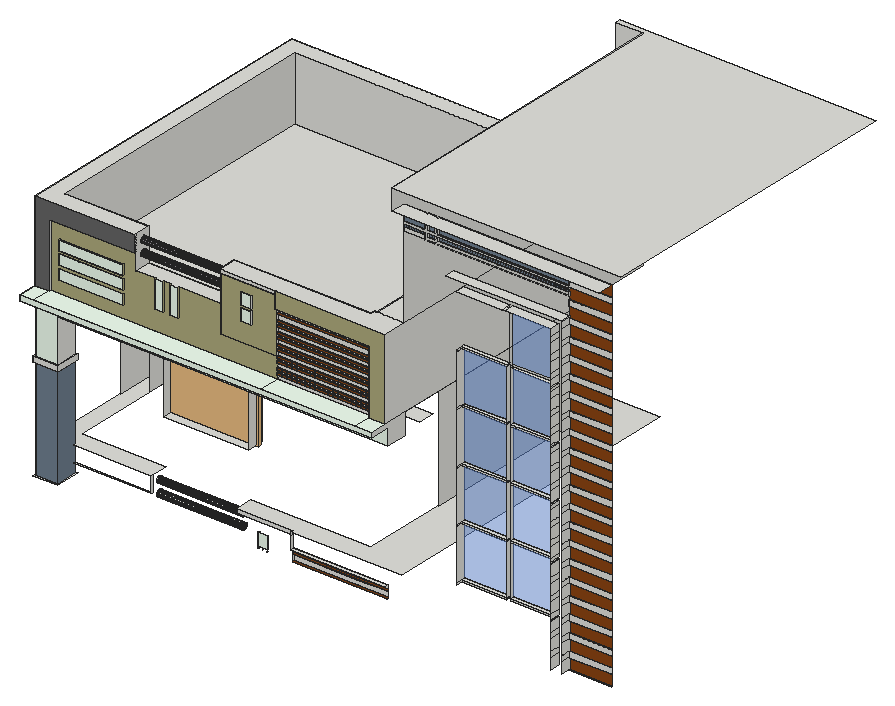
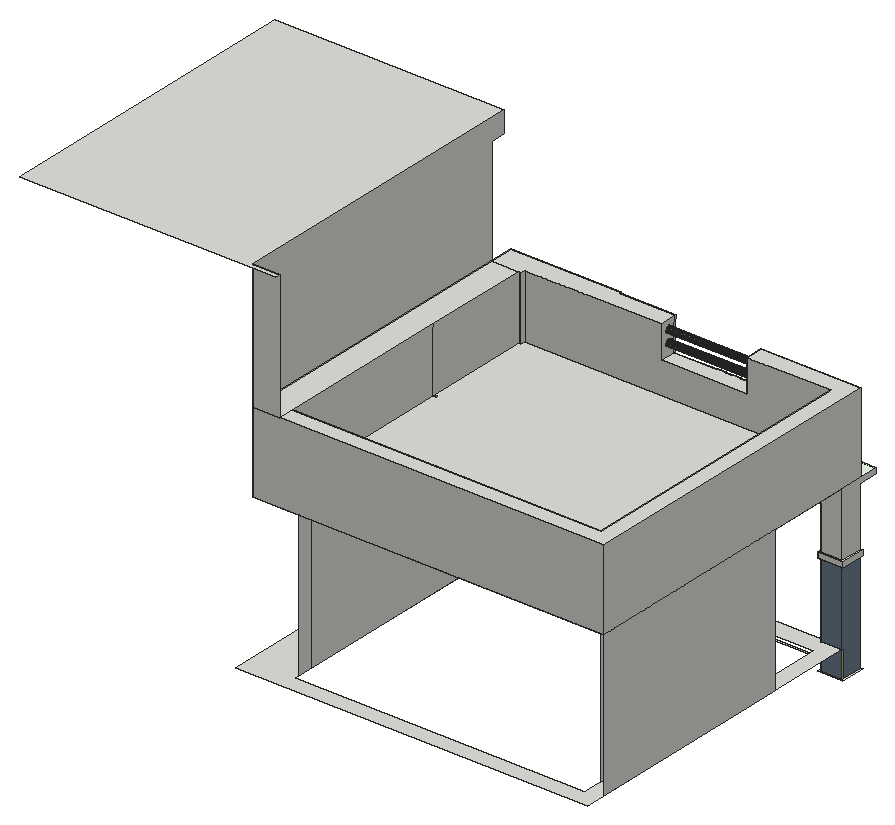
# SketchUp Ruby script. Lengths in inches.
U = 1.inch
M = Sketchup.active_model
def pt(a) = Geom::Point3d.new(a.map { |v| v * U })
def face(e, loops, mat)
  f = e.add_face(loops[0].map { |a| pt(a) })
  loops[1..].each { |l| e.add_face(l.map { |a| pt(a) }).erase! }
  f.material = f.back_material = mat if mat
  f
end
# faces: each face lists its corners as indices into pts; further lists are holes
def faces(e, pts, list, mat = nil) = list.each { |f| face(e, (f[0].is_a?(Array) ? f : [f]).map { |l| l.map { |i| pts[i] } }, mat) }
# xy, xz, yz: faces in a plane at the given z, y or x. An outline is a flat list of corners, or four numbers for a rectangle; further outlines are holes
def ring(l) = l.size == 4 ? [[l[0], l[1]], [l[2], l[1]], [l[2], l[3]], [l[0], l[3]]] : l.each_slice(2).to_a
def flat(e, list, mat, &to3) = list.each { |f| face(e, (f[0].is_a?(Array) ? f : [f]).map { |l| ring(l).map { |u, v| to3.(u, v) } }, mat) }
def xy(e, z, list, mat = nil) = flat(e, list, mat) { |x, y| [x, y, z] }
def xz(e, y, list, mat = nil) = flat(e, list, mat) { |x, z| [x, y, z] }
def yz(e, x, list, mat = nil) = flat(e, list, mat) { |y, z| [x, y, z] }
def lines(e, pts, list) = list.each { |a, b| e.add_line(pt(pts[a]), pt(pts[b])) }
# prism: a flat outline (further loops are holes) pulled along v
def prism(e, loops, v, mat = nil)
  f = face(e, loops, mat); d = Geom::Vector3d.new(v.map { |x| x * U })
  f.pushpull(f.normal.samedirection?(d) ? d.length : -d.length)
end
def box(e, o, s, mat = nil) = prism(e, [[o, [o[0] + s[0], o[1], o[2]], [o[0] + s[0], o[1] + s[1], o[2]], [o[0], o[1] + s[1], o[2]]]], [0, 0, s[2]], mat)
def at(x, y, z, deg = 0) = Geom::Transformation.translation(pt([x, y, z])) * Geom::Transformation.rotation(ORIGIN, Z_AXIS, deg.degrees)
def axes(o, x, y, z) = Geom::Transformation.new([*x, 0, *y, 0, *z, 0, *pt(o).to_a, 1])
def part(name) = M.definitions.add(name)
# library, detail: a bought-in or finely detailed component or shape, given as its bounding box
def library(name, o, s) = part(name).tap { |d| box(d.entities, o, s) }
def detail(e, o, s) = box(e.add_group.entities, o, s)
def put(e, d, t, mat = nil) = e.add_instance(d, t).tap { |i| i.material = mat if mat }
def group(e, t, mat = nil) = e.add_group.tap { |g| g.transformation = t; g.material = mat if mat }.entities
root = M.entities
M.materials.add("Teddy_Bracelet").color = [145, 141, 147]
M.materials.add("[0043_SaddleBrown]").color = [139, 69, 19]
M.materials.add("[0047_Khaki]").color = [198, 190, 116]
M.materials.add("[0048_PaleGoldenrod]1").color = [175, 171, 125]
M.materials.add("[0066_Honeydew]").color = [240, 255, 240]
M.materials.add("[0111_SlateGray]").color = [112, 128, 144]
M.materials.add("[0134_DimGray]").color = [102, 102, 102]
M.materials.add("[Translucent Glass Blue]").color = [100, 149, 237]
M.materials["[Translucent Glass Blue]"].alpha = 0.5
c1 = library("Double-hung window 69 in. x 58 in. triple row with mullions",[0,0,-2.625],[62,58,3.625])
c2 = part("Double-hung window assembly")
put(c2.entities,c1,axes([2046.74,517.98,-571.2],[-3.288,0,0],[0,0,3.072],[0,2.4,0]))
xy(root,149,[[136.36,47.5,172.375,48],[172.375,47.5,189.375,48]])
xy(root,149.3,[[291.09,47.5,315.09,48]])
xy(root,149.33,[[116.69,47,122.32,47.5]])
xy(root,150,[[[0,35.4375,14,49.4375],[1,36.4375,13,48.4375]],[1,36.4375,13,48.4375]])
xy(root,150,[[136.36,47.5,172.375,48],[172.375,47.5,189.375,48]],"[0043_SaddleBrown]")
xy(root,150.64,[[116.69,47,122.32,47.5]])
xy(root,153,[[136.36,47.5,172.375,48],[172.375,47.5,189.375,48]])
xy(root,154,[[136.36,47.5,172.375,48],[172.375,47.5,189.375,48]],"[0043_SaddleBrown]")
xy(root,155.45,[[291.09,47.5,315.09,48]])
xy(root,156,[[136.36,45.9375,189.375,48],[9.125,47,57.01,48]])
xy(root,157.33,[[116.69,47,122.32,47.5]])
xy(root,158.61,[[291.09,47.5,315.09,48]])
xy(root,162,[[25,95.625,73,104.625]])
xy(root,163,[[104.95,47,136.36,47.5]])
xy(root,164.77,[[291.09,47.5,315.09,48]])
xy(root,165,[[136.36,45.9375,198.375,45.9375,198.375,227.1875,1,227.1875,1,47,57.01,47,57.01,57,10,57,10,218.1875,172.375,218.1875,172.375,57,104.95,57,104.95,47,136.36,47]])
xy(root,167.92,[[291.09,47.5,315.09,48]])
xy(root,173.4,[[232.02,46,257.55,48],[259.55,46,285.09,48]])
xy(root,174.08,[[291.09,47.5,315.09,48]])
xy(root,174.4,[[232.02,46,257.55,48],[259.55,46,285.09,48]])
xy(root,177.23,[[291.09,47.5,315.09,48]])
xy(root,183.39,[[291.09,47.5,315.09,48]])
xy(root,186.55,[[291.09,47.5,315.09,48]])
xy(root,192.7,[[291.09,47.5,315.09,48]])
xy(root,195.86,[[291.09,47.5,315.09,48]])
xy(root,202.01,[[291.09,47.5,315.09,48]])
xy(root,202.68,[[232.02,46,257.55,48],[259.55,46,285.09,48]])
xy(root,203.68,[[232.02,46,257.55,47.8125],[259.55,46,285.09,48]])
xy(root,205.17,[[291.09,47.5,315.09,48]])
xy(root,207,[[0,35.4375,14,36.4375],[0,36.4375,1,49.4375],[1,36.4375,13,48.4375],[13,36.4375,14,49.4375],[1,48.4375,13,49.4375]])
xy(root,208.1875,[[25,95.625,73,104.625]])
xy(root,210,[[[0,35.4375,14,49.4375],[1,36.4375,13,48.4375]],[1,36.4375,13,48.4375],[133.23,95.625,169.23,104.625]])
xy(root,211.32,[[291.09,47.5,315.09,48]])
xy(root,214.48,[[291.09,47.5,315.09,48]])
xy(root,220.64,[[291.09,47.5,315.09,48]])
xy(root,223.79,[[291.09,47.5,315.09,48]])
xy(root,229.95,[[291.09,47.5,315.09,48]])
xy(root,231.95,[[232.02,46,257.55,47.8125],[259.55,46,285.09,48]])
xy(root,232.95,[[232.02,46,257.55,48],[259.55,46,285.09,48]])
xy(root,233.11,[[291.09,47.5,315.09,48]])
xy(root,234,[[13,36.4375,198.375,48.4375]])
xy(root,239.26,[[291.09,47.5,315.09,48]])
xy(root,242.42,[[291.09,47.5,315.09,48]])
xy(root,243,[[1,24.875,198.375,36.4375]],"[0066_Honeydew]")
xy(root,246,[[189.375,34.375,189.375,36.4375,9.125,36.4375,9.125,35.4375,1,35.4375,1,48.4375,198.375,48.4375,198.375,34.375],[1,48.4375,172.375,95.625],[172.375,48.4375,198.375,95.625],[1,95.625,172.375,95.625,172.375,104.625,10,104.625,10,206.625,172.375,206.625,172.375,215.625,1,215.625],[172.375,95.625,181.375,104.625],
  [181.375,95.625,198.375,104.625],[10,104.625,172.375,206.625],[172.375,104.625,181.375,215.625],[181.375,104.625,198.375,215.625]])
xy(root,246,[[1,24.875,9.125,35.4375],[9.125,24.875,136.36,36.4375],[136.36,24.875,189.375,36.4375],[189.375,24.875,198.375,34.375]],"[0066_Honeydew]")
xy(root,248.5,[[136.36,35.9375,172.375,36.4375],[172.375,35.9375,189.375,36.4375]])
xy(root,248.57,[[291.09,47.5,315.09,48]])
xy(root,249.5,[[136.36,35.9375,172.375,36.4375],[172.375,35.9375,189.375,36.4375]],"[0043_SaddleBrown]")
xy(root,251,[[136.36,35.9375,172.375,36.4375],[172.375,35.9375,189.375,36.4375]])
xy(root,251.73,[[291.09,47.5,315.09,48]])
xy(root,252,[[136.36,35.9375,172.375,36.4375],[172.375,35.9375,189.375,36.4375]],"[0043_SaddleBrown]")
xy(root,253.11,[[14.32,35.9375,50.14,36.4375]],"[0048_PaleGoldenrod]1")
xy(root,254.5,[[136.36,35.9375,172.375,36.4375],[172.375,35.9375,189.375,36.4375]])
xy(root,255,[[10,45.4375,181.625,45.4375,181.625,48,183,48,183,107.1875,181.375,107.1875,181.375,108,183,108,183,206.625,10,206.625],[181.375,107.1875,183,108]])
xy(root,255.5,[[136.36,35.9375,172.375,36.4375],[172.375,35.9375,189.375,36.4375]],"[0043_SaddleBrown]")
xy(root,257,[[136.36,35.9375,172.375,36.4375],[172.375,35.9375,189.375,36.4375]])
xy(root,257.375,[[68.2,35.9375,72.45,36.4375],[76.51,35.9375,80.76,36.4375]],"[0048_PaleGoldenrod]1")
xy(root,257.8125,[[104.95,35.9375,136.36,36.4375]])
xy(root,257.88,[[291.09,47.5,315.09,48]])
xy(root,258,[[136.36,35.9375,172.375,36.4375],[172.375,35.9375,189.375,36.4375]],"[0043_SaddleBrown]")
xy(root,258.61,[[14.32,35.9375,50.14,36.4375]],"[0048_PaleGoldenrod]1")
xy(root,260.5,[[136.36,35.9375,172.375,36.4375],[172.375,35.9375,189.375,36.4375]])
xy(root,260.8,[[14.32,35.9375,50.14,36.4375]],"[0048_PaleGoldenrod]1")
xy(root,261.04,[[291.09,47.5,315.09,48]])
xy(root,261.23,[[232.02,46,257.55,48],[259.55,46,285.09,48]])
xy(root,261.5,[[136.36,35.9375,172.375,36.4375],[172.375,35.9375,189.375,36.4375]],"[0043_SaddleBrown]")
xy(root,262.23,[[232.02,46,257.55,48],[259.55,46,285.09,48]])
xy(root,263,[[136.36,35.9375,172.375,36.4375],[172.375,35.9375,189.375,36.4375]])
xy(root,264,[[136.36,35.9375,172.375,36.4375],[172.375,35.9375,189.375,36.4375]],"[0043_SaddleBrown]")
xy(root,266.3,[[14.32,35.9375,50.14,36.4375]],"[0048_PaleGoldenrod]1")
xy(root,266.5,[[136.36,35.9375,172.375,36.4375],[172.375,35.9375,189.375,36.4375]])
xy(root,267.19,[[291.09,47.5,315.09,48]])
xy(root,267.5,[[136.36,35.9375,172.375,36.4375],[172.375,35.9375,189.375,36.4375]],"[0043_SaddleBrown]")
xy(root,268.05,[[14.32,35.9375,50.14,36.4375]],"[0048_PaleGoldenrod]1")
xy(root,268.64,[[116.69,35.4375,122.32,35.9375]])
xy(root,269,[[136.36,35.9375,172.375,36.4375],[172.375,35.9375,189.375,36.4375]])
xy(root,270,[[136.36,35.9375,172.375,36.4375],[172.375,35.9375,189.375,36.4375]],"[0043_SaddleBrown]")
xy(root,270.35,[[291.09,47.5,315.09,48]])
xy(root,272.5,[[136.36,35.9375,172.375,36.4375],[172.375,35.9375,189.375,36.4375]])
xy(root,272.6875,[[68.2,35.9375,72.45,35.9375,72.45,36.4375,76.51,36.4375,76.51,35.9375,80.76,35.9375,80.76,36.4375,104.95,36.4375,104.95,45.4375,57.01,45.4375,57.01,36.4375,68.2,36.4375]])
xy(root,273.5,[[136.36,35.9375,172.375,36.4375],[172.375,35.9375,189.375,36.4375]],"[0043_SaddleBrown]")
xy(root,273.55,[[14.32,35.9375,50.14,36.4375]],"[0048_PaleGoldenrod]1")
xy(root,275,[[136.36,35.9375,172.375,36.4375],[172.375,35.9375,189.375,36.4375]])
xy(root,275.33,[[116.69,35.4375,122.32,35.9375]])
xy(root,276,[[136.36,35.9375,172.375,36.4375],[172.375,35.9375,189.375,36.4375]],"[0043_SaddleBrown]")
xy(root,276.51,[[291.09,47.5,315.09,48]])
xy(root,276.64,[[116.69,35.4375,122.32,35.9375]])
xy(root,279,[[136.36,35.9375,172.375,36.4375],[172.375,35.9375,189.375,36.4375]])
xy(root,279.66,[[291.09,47.5,315.09,48]])
xy(root,280,[[136.36,35.9375,172.375,36.4375],[172.375,35.9375,189.375,36.4375]],"[0043_SaddleBrown]")
xy(root,282,[[136.36,34.375,189.375,36.4375],[9.125,35.4375,57.01,36.4375]])
xy(root,283.33,[[116.69,35.4375,122.32,35.9375]])
xy(root,285.82,[[291.09,47.5,315.09,48]])
xy(root,288.98,[[291.09,47.5,315.09,48]])
xy(root,289,[[104.95,35.4375,136.36,35.9375]])
xy(root,290.51,[[232.02,46,257.55,48],[259.55,46,285.09,48]])
xy(root,291,[[136.36,34.375,198.375,34.375,198.375,48,181.625,48,181.625,45.4375,104.95,45.4375,104.95,35.4375,136.36,35.4375],[1,35.4375,57.01,35.4375,57.01,45.4375,10,45.4375,10,206.625,183,206.625,183,215.625,1,215.625],[183,48,198.375,215.625]])
xy(root,291.51,[[232.02,46,257.55,48]])
xy(root,295.13,[[291.09,47.5,315.09,48]])
xy(root,298.29,[[291.09,47.5,315.09,48]])
xy(root,304.44,[[291.09,47.5,315.09,48]])
xy(root,307.6,[[291.09,47.5,315.09,48]])
xy(root,313.75,[[291.09,47.5,315.09,48]])
xy(root,316.91,[[291.09,47.5,315.09,48]])
xy(root,320.78,[[232.02,42.5,257.55,48],[257.55,42.5,259.55,46],[259.55,42.5,285.09,48]])
xy(root,323.06,[[291.09,47.5,315.09,48]])
xy(root,326.22,[[291.09,47.5,315.09,48]])
xy(root,326.78,[[226.02,42.5,291.09,48]])
xy(root,332.375,[[291.09,47.5,315.09,48]])
xy(root,335.53,[[291.09,47.5,315.09,48]])
xy(root,337.1875,[[212.0625,47.5,215.8125,48],[217.8125,47.5,291.09,48]])
xy(root,339.1875,[[212.0625,47.5,215.8125,48],[217.8125,47.5,291.09,48]])
xy(root,340.5,[[198.375,47.5,210.0625,48],[212.0625,47.5,215.8125,48],[217.8125,47.5,291.09,48]])
xy(root,341.6875,[[291.09,47.5,315.09,48]])
xy(root,342.5,[[198.375,47.5,210.0625,48],[212.0625,47.5,215.8125,48],[217.8125,47.5,291.09,48]])
xy(root,344.85,[[291.09,47.5,315.09,48]])
xy(root,351,[[198.375,39,198.375,48,210.0625,48,210.0625,47.5,212.0625,47.5,212.0625,48,215.8125,48,215.8125,47.5,217.8125,47.5,217.8125,48,315.09,48,315.09,39]])
xy(root,363,[[198.375,39,327,39,327,218.1875,183,218.1875,183,215.625,198.375,215.625]])
xz(root,24.875,[[1,243,198.375,246]],"[0066_Honeydew]")
xz(root,34.375,[[189.375,246,198.375,246,198.375,291,136.36,291,136.36,282,189.375,282]],"[0048_PaleGoldenrod]1")
xz(root,35.4375,[[0,207,14,210],[104.95,289,136.36,291]])
xz(root,35.4375,[[116.69,268.64,122.32,275.33],[116.69,276.64,122.32,283.33]],"[0066_Honeydew]")
xz(root,35.4375,[[1,246,9.125,246,9.125,282,57.01,282,57.01,291,1,291]],"[0134_DimGray]")
xz(root,35.9375,[[136.36,248.5,189.375,249.5],[136.36,251,189.375,252],[136.36,254.5,189.375,255.5],[136.36,257,189.375,258],[136.36,260.5,189.375,261.5],
  [136.36,263,189.375,264],[136.36,266.5,189.375,267.5],[136.36,269,189.375,270],[136.36,272.5,189.375,273.5],[136.36,275,189.375,276],
  [136.36,279,189.375,280]],"[0043_SaddleBrown]")
xz(root,35.9375,[[[104.95,257.8125,136.36,289],[116.69,276.64,122.32,283.33],[116.69,268.64,122.32,275.33]]],"[0048_PaleGoldenrod]1")
xz(root,35.9375,[[14.32,253.11,50.14,258.61],[68.2,257.375,72.45,272.6875],[76.51,257.375,80.76,272.6875],[14.32,260.8,50.14,266.3],[14.32,268.05,50.14,273.55]],"[0066_Honeydew]")
xz(root,36.4375,[[136.36,246,189.375,248.5],[136.36,249.5,189.375,251],[136.36,252,189.375,254.5],[136.36,255.5,189.375,257],[136.36,258,189.375,260.5],
  [136.36,261.5,189.375,263],[136.36,264,189.375,266.5],[136.36,267.5,189.375,269],[136.36,270,189.375,272.5],[136.36,273.5,189.375,275],
  [136.36,276,189.375,279],[136.36,280,189.375,282]])
xz(root,36.4375,[[[9.125,246,136.36,246,136.36,257.8125,104.95,257.8125,104.95,272.6875,80.76,272.6875,80.76,257.375,76.51,257.375,76.51,272.6875,72.45,272.6875,72.45,257.375,68.2,257.375,68.2,272.6875,57.01,272.6875,57.01,282,9.125,282],[14.32,268.05,50.14,273.55],[14.32,260.8,50.14,266.3],[14.32,253.11,50.14,258.61]]],"[0048_PaleGoldenrod]1")
xz(root,36.4375,[[1,210,13,210,13,234,198.375,234,198.375,243,1,243]],"[0066_Honeydew]")
xz(root,36.4375,[[1,150,13,207]],"[0111_SlateGray]")
xz(root,45.4375,[[10,255,10,291,57.01,291,57.01,272.6875,104.95,272.6875,104.95,291,181.625,291,181.625,255]])
xz(root,46,[[232.02,173.4,257.55,174.4],[259.55,173.4,285.09,174.4],[232.02,202.68,257.55,203.68],[259.55,202.68,285.09,203.68],[232.02,231.95,257.55,232.95],
  [259.55,231.95,285.09,232.95],[232.02,261.23,257.55,262.23],[259.55,261.23,285.09,262.23],[232.02,290.51,257.55,291.51]])
xz(root,47,[[104.95,163,136.36,165]])
xz(root,47,[[116.69,150.64,122.32,157.33]],"[0066_Honeydew]")
xz(root,47.5,[[291.09,155.45,315.09,158.61],[291.09,164.77,315.09,167.92],[291.09,174.08,315.09,177.23],[291.09,183.39,315.09,186.55],[291.09,192.7,315.09,195.86],
  [291.09,202.01,315.09,205.17],[291.09,211.32,315.09,214.48],[291.09,220.64,315.09,223.79],[291.09,229.95,315.09,233.11],[291.09,239.26,315.09,242.42],
  [291.09,248.57,315.09,251.73],[291.09,257.88,315.09,261.04],[291.09,267.19,315.09,270.35],[291.09,276.51,315.09,279.66],[291.09,285.82,315.09,288.98],
  [291.09,295.13,315.09,298.29],[291.09,304.44,315.09,307.6],[291.09,313.75,315.09,316.91],[291.09,323.06,315.09,326.22],[291.09,332.375,315.09,335.53],
  [291.09,341.6875,315.09,344.85]])
xz(root,47.5,[[136.36,149,189.375,150],[136.36,153,189.375,154]],"[0043_SaddleBrown]")
xz(root,47.8125,[[232.02,203.68,257.55,231.95]],"[Translucent Glass Blue]")
xz(root,48,[[136.36,150,189.375,153],[136.36,154,189.375,156],[181.625,255,183,291],[198.375,337.1875,210.0625,339.1875]])
xz(root,48,[[291.09,149.3,315.09,155.45],[291.09,158.61,315.09,164.77],[291.09,167.92,315.09,174.08],[291.09,177.23,315.09,183.39],[291.09,186.55,315.09,192.7],
  [291.09,195.86,315.09,202.01],[291.09,205.17,315.09,211.32],[291.09,214.48,315.09,220.64],[291.09,223.79,315.09,229.95],[291.09,233.11,315.09,239.26],
  [291.09,242.42,315.09,248.57],[291.09,251.73,315.09,257.88],[291.09,261.04,315.09,267.19],[291.09,270.35,315.09,276.51],[291.09,279.66,315.09,285.82],
  [291.09,288.98,315.09,295.13],[291.09,298.29,315.09,304.44],[291.09,307.6,315.09,313.75],[291.09,316.91,315.09,323.06],[291.09,326.22,315.09,332.375],
  [291.09,335.53,315.09,341.6875],[291.09,344.85,315.09,351]],"[0043_SaddleBrown]")
xz(root,48,[[198.375,339.1875,210.0625,340.5],[212.0625,339.1875,215.8125,340.5],[217.8125,339.1875,291.09,340.5],[198.375,342.5,210.0625,351],[212.0625,342.5,215.8125,351],
  [217.8125,342.5,291.09,351]],"[0111_SlateGray]")
xz(root,48,[[232.02,174.4,257.55,202.68],[259.55,174.4,285.09,202.68],[259.55,203.68,285.09,231.95],[232.02,232.95,257.55,261.23],[259.55,232.95,285.09,261.23],
  [232.02,262.23,257.55,290.51],[259.55,262.23,285.09,290.51],[259.55,291.51,285.09,320.78]],"[Translucent Glass Blue]")
xz(root,48.4375,[[1,210,1,246,198.375,246,198.375,234,13,234,13,210]])
xz(root,48.4375,[[1,150,13,207]],"[0111_SlateGray]")
xz(root,49.4375,[[0,207,14,210]])
xz(root,206.625,[[10,255,183,291]])
xz(root,215.625,[[1,246,198.375,291],[183,291,198.375,363]])
yz(root,0,[[35.4375,207,49.4375,210]])
yz(root,1,[[95.625,165,215.625,246],[36.4375,210,36.4375,243,24.875,243,24.875,246,48.4375,246,48.4375,210],[35.4375,246,215.625,291]])
yz(root,1,[[47,150,48.4375,165]],"[0047_Khaki]")
yz(root,1,[[36.4375,150,36.4375,207,48.4375,207,48.4375,165,47,165,47,150]],"[0111_SlateGray]")
yz(root,9.125,[[35.4375,246,36.4375,282]])
yz(root,10,[[104.625,165,206.625,246],[45.4375,255,206.625,291]])
yz(root,13,[[36.4375,210,48.4375,234]])
yz(root,13,[[36.4375,150,48.4375,207]],"[0111_SlateGray]")
yz(root,14,[[35.4375,207,49.4375,210]])
yz(root,14.32,[[35.9375,253.11,36.4375,258.61],[35.9375,260.8,36.4375,266.3],[35.9375,268.05,36.4375,273.55]],"[0048_PaleGoldenrod]1")
yz(root,25,[[95.625,162,104.625,208.1875]])
yz(root,50.14,[[35.9375,253.11,36.4375,258.61],[35.9375,260.8,36.4375,266.3],[35.9375,268.05,36.4375,273.55]],"[0048_PaleGoldenrod]1")
yz(root,57.01,[[47,156,48,165],[[36.4375,272.6875,45.4375,291],[41.02,284.88,40.58,284.94,40.18,285.11,39.83,285.38,39.56,285.73,39.39,286.13,39.33,286.57,39.39,287.01,39.56,287.41,39.83,287.76,40.18,288.03,40.58,288.2,41.02,288.26,41.46,288.2,41.86,288.03,42.21,287.76,42.48,287.41,42.65,287.01,42.71,286.57,42.65,286.13,42.48,285.73,42.21,285.38,41.86,285.11,41.46,284.94],[41.02,278.13,40.58,278.19,40.18,278.36,39.83,278.63,39.56,278.98,39.39,279.38,39.33,279.82,39.39,280.26,39.56,280.66,39.83,281.01,40.18,281.28,40.58,281.45,41.02,281.51,41.46,281.45,41.86,281.28,42.21,281.01,42.48,280.66,42.65,280.26,42.71,279.82,42.65,279.38,42.48,278.98,42.21,278.63,41.86,278.36,41.46,278.19]],[35.4375,282,36.4375,291]])
yz(root,68.2,[[35.9375,257.375,36.4375,272.6875]],"[0048_PaleGoldenrod]1")
yz(root,72.45,[[35.9375,257.375,36.4375,272.6875]],"[0048_PaleGoldenrod]1")
yz(root,73,[[95.625,162,104.625,208.1875]])
yz(root,76.51,[[35.9375,257.375,36.4375,272.6875]],"[0048_PaleGoldenrod]1")
yz(root,80.76,[[35.9375,257.375,36.4375,272.6875]],"[0048_PaleGoldenrod]1")
yz(root,104.95,[[47,163,48,165],[35.9375,257.8125,36.4375,272.6875],[35.9375,272.6875,36.4375,289],[[36.4375,272.6875,45.4375,291],[41.02,284.88,41.46,284.94,41.86,285.11,42.21,285.38,42.48,285.73,42.65,286.13,42.71,286.57,42.65,287.01,42.48,287.41,42.21,287.76,41.86,288.03,41.46,288.2,41.02,288.26,40.58,288.2,40.18,288.03,39.83,287.76,39.56,287.41,39.39,287.01,39.33,286.57,39.39,286.13,39.56,285.73,39.83,285.38,40.18,285.11,40.58,284.94],[41.02,278.13,41.46,278.19,41.86,278.36,42.21,278.63,42.48,278.98,42.65,279.38,42.71,279.82,42.65,280.26,42.48,280.66,42.21,281.01,41.86,281.28,41.46,281.45,41.02,281.51,40.58,281.45,40.18,281.28,39.83,281.01,39.56,280.66,39.39,280.26,39.33,279.82,39.39,279.38,39.56,278.98,39.83,278.63,40.18,278.36,40.58,278.19]],[35.4375,289,36.4375,291]])
yz(root,116.69,[[47,150.64,47.5,157.33],[35.4375,268.64,35.9375,275.33],[35.4375,276.64,35.9375,283.33]])
yz(root,122.32,[[47,150.64,47.5,157.33],[35.4375,268.64,35.9375,275.33],[35.4375,276.64,35.9375,283.33]])
yz(root,136.36,[[47.5,150,48,153],[47.5,154,48,156],[45.9375,156,47.5,163],[45.9375,163,47,165],[35.9375,258,36.4375,260.5],
  [35.9375,261.5,36.4375,263],[35.9375,264,36.4375,266.5],[35.9375,267.5,36.4375,269],[35.9375,270,36.4375,272.5],[35.9375,273.5,36.4375,275],
  [35.9375,276,36.4375,279],[35.9375,280,36.4375,282],[34.375,282,35.9375,289],[34.375,289,35.4375,291]])
yz(root,136.36,[[35.9375,248.5,36.4375,249.5],[35.9375,251,36.4375,252],[35.9375,254.5,36.4375,255.5],[35.9375,257,36.4375,257.8125]],"[0043_SaddleBrown]")
yz(root,172.375,[[104.625,165,206.625,246],[206.625,165,215.625,246]])
yz(root,181.375,[[107.1875,246,108,255]])
yz(root,181.625,[[45.4375,255,48,291]])
yz(root,183,[[48,255,108,291],[108,255,206.625,291]])
yz(root,189.375,[[34.375,246,34.375,282,36.4375,282,36.4375,280,35.9375,280,35.9375,279,36.4375,279,36.4375,276,35.9375,276,35.9375,275,36.4375,275,36.4375,273.5,35.9375,273.5,35.9375,272.5,36.4375,272.5,36.4375,270,35.9375,270,35.9375,269,36.4375,269,36.4375,267.5,35.9375,267.5,35.9375,266.5,36.4375,266.5,36.4375,264,35.9375,264,35.9375,263,36.4375,263,36.4375,261.5,35.9375,261.5,35.9375,260.5,36.4375,260.5,36.4375,258,35.9375,258,35.9375,257,36.4375,257,36.4375,255.5,35.9375,255.5,35.9375,254.5,36.4375,254.5,36.4375,252,35.9375,252,35.9375,251,36.4375,251,36.4375,249.5,35.9375,249.5,35.9375,248.5,36.4375,248.5,36.4375,246]])
yz(root,198.375,[[36.4375,234,48.4375,234,48.4375,246,24.875,246,24.875,243,36.4375,243],[34.375,246,215.625,291],[48,291,48,340.5,47.5,340.5,47.5,342.5,48,342.5,48,351,39,351,39,363,215.625,363,215.625,291]])
yz(root,210.0625,[[47.5,337.1875,48,339.1875],[47.5,339.1875,48,340.5],[47.5,342.5,48,351]])
yz(root,212.0625,[[47.5,339.1875,48,340.5],[47.5,342.5,48,351]])
yz(root,215.8125,[[47.5,339.1875,48,340.5],[47.5,342.5,48,351]])
yz(root,217.8125,[[47.5,339.1875,48,340.5],[47.5,342.5,48,351]])
yz(root,232.02,[[42.5,173.4,46,174.4],[42.5,174.4,48,202.68],[42.5,202.68,46,203.68],[42.5,203.68,47.8125,231.95],[42.5,231.95,46,232.95],
  [42.5,232.95,48,261.23],[42.5,261.23,46,262.23],[42.5,262.23,48,290.51],[42.5,290.51,46,291.51]])
yz(root,257.55,[[46,174.4,48,202.68],[46,203.68,47.8125,231.95],[46,232.95,48,261.23],[46,262.23,48,290.51]])
yz(root,259.55,[[46,174.4,48,202.68],[46,203.68,48,231.95],[46,232.95,48,261.23],[46,262.23,48,290.51]])
yz(root,285.09,[[42.5,149.3,48,155.45],[42.5,155.45,48,158.61],[42.5,158.61,48,164.77],[42.5,164.77,48,167.92],[42.5,167.92,48,173.4],
  [42.5,173.4,46,174.08],[42.5,174.08,46,174.4],[42.5,174.4,48,177.23],[42.5,177.23,48,183.39],[42.5,183.39,48,186.55],
  [42.5,186.55,48,192.7],[42.5,192.7,48,195.86],[42.5,195.86,48,202.01],[42.5,202.01,48,202.68],[42.5,202.68,46,203.68],
  [42.5,203.68,48,205.17],[42.5,205.17,48,211.32],[42.5,211.32,48,214.48],[42.5,214.48,48,220.64],[42.5,220.64,48,223.79],
  [42.5,223.79,48,229.95],[42.5,229.95,48,231.95],[42.5,231.95,46,232.95],[42.5,232.95,48,233.11],[42.5,233.11,48,239.26],
  [42.5,239.26,48,242.42],[42.5,242.42,48,248.57],[42.5,248.57,48,251.73],[42.5,251.73,48,257.88],[42.5,257.88,48,261.04],
  [42.5,261.04,48,261.23],[42.5,261.23,46,262.23],[42.5,262.23,48,267.19],[42.5,267.19,48,270.35],[42.5,270.35,48,276.51],
  [42.5,276.51,48,279.66],[42.5,279.66,48,285.82],[42.5,285.82,48,288.98],[42.5,288.98,48,290.51],[42.5,290.51,46,291.51],
  [42.5,291.51,48,295.13],[42.5,295.13,48,298.29],[42.5,298.29,48,304.44],[42.5,304.44,48,307.6],[42.5,307.6,48,313.75],
  [42.5,313.75,48,316.91],[42.5,316.91,48,320.78]])
yz(root,291.09,[[42.5,149.3,48,155.45],[42.5,155.45,47.5,158.61],[42.5,158.61,48,164.77],[42.5,164.77,47.5,167.92],[42.5,167.92,48,174.08],
  [42.5,174.08,47.5,177.23],[42.5,177.23,48,183.39],[42.5,183.39,47.5,186.55],[42.5,186.55,48,192.7],[42.5,192.7,47.5,195.86],
  [42.5,195.86,48,202.01],[42.5,202.01,47.5,205.17],[42.5,205.17,48,211.32],[42.5,211.32,47.5,214.48],[42.5,214.48,48,220.64],
  [42.5,220.64,47.5,223.79],[42.5,223.79,48,229.95],[42.5,229.95,47.5,233.11],[42.5,233.11,48,239.26],[42.5,239.26,47.5,242.42],
  [42.5,242.42,48,248.57],[42.5,248.57,47.5,251.73],[42.5,251.73,48,257.88],[42.5,257.88,47.5,261.04],[42.5,261.04,48,267.19],
  [42.5,267.19,47.5,270.35],[42.5,270.35,48,276.51],[42.5,276.51,47.5,279.66],[42.5,279.66,48,285.82],[42.5,285.82,47.5,288.98],
  [42.5,288.98,48,295.13],[42.5,295.13,47.5,298.29],[42.5,298.29,48,304.44],[42.5,304.44,47.5,307.6],[42.5,307.6,48,313.75],
  [42.5,313.75,47.5,316.91],[42.5,316.91,48,323.06],[42.5,323.06,47.5,326.22],[42.5,326.22,48,326.78],[47.5,332.375,48,335.53],
  [47.5,337.1875,48,339.1875],[47.5,340.5,48,341.6875],[47.5,342.5,48,344.85]])
p = [[57.01,52.14,152.19],[57.01,52.58,152.13],[104.95,52.58,152.13],[104.95,52.14,152.19],[57.01,53.02,152.19],[104.95,53.02,152.19],
  [57.01,51.74,152.36],[104.95,51.74,152.36],[57.01,53.43,152.36],[104.95,53.43,152.36],[57.01,51.39,152.63],[104.95,51.39,152.63],
  [57.01,53.77,152.63],[104.95,53.77,152.63],[57.01,51.12,152.98],[104.95,51.12,152.98],[57.01,54.04,152.98],[104.95,54.04,152.98],
  [57.01,50.95,153.38],[104.95,50.95,153.38],[57.01,54.21,153.38],[104.95,54.21,153.38],[57.01,50.89,153.82],[104.95,50.89,153.82],
  [57.01,54.27,153.82],[104.95,54.27,153.82],[57.01,50.95,154.26],[104.95,50.95,154.26],[57.01,54.21,154.26],[104.95,54.21,154.26],
  [57.01,51.12,154.66],[104.95,51.12,154.66],[57.01,54.04,154.66],[104.95,54.04,154.66],[57.01,51.39,155.01],[104.95,51.39,155.01],
  [57.01,53.77,155.01],[104.95,53.77,155.01],[57.01,51.74,155.28],[104.95,51.74,155.28],[57.01,53.43,155.28],[104.95,53.43,155.28],
  [57.01,52.14,155.45],[104.95,52.14,155.45],[57.01,53.02,155.45],[104.95,53.02,155.45],[57.01,52.58,155.51],[104.95,52.58,155.51],
  [57.01,51.74,159.11],[57.01,52.14,158.94],[104.95,52.14,158.94],[104.95,51.74,159.11],[57.01,52.58,158.88],[104.95,52.58,158.88],
  [57.01,53.02,158.94],[104.95,53.02,158.94],[57.01,53.43,159.11],[104.95,53.43,159.11],[57.01,51.39,159.38],[104.95,51.39,159.38],
  [57.01,53.77,159.38],[104.95,53.77,159.38],[57.01,51.12,159.73],[104.95,51.12,159.73],[57.01,54.04,159.73],[104.95,54.04,159.73],
  [57.01,50.95,160.13],[104.95,50.95,160.13],[57.01,54.21,160.13],[104.95,54.21,160.13],[57.01,50.89,160.57],[104.95,50.89,160.57],
  [57.01,54.27,160.57],[104.95,54.27,160.57],[57.01,50.95,161.01],[104.95,50.95,161.01],[57.01,54.21,161.01],[104.95,54.21,161.01],
  [57.01,51.12,161.41],[104.95,51.12,161.41],[57.01,54.04,161.41],[104.95,54.04,161.41],[57.01,51.39,161.76],[104.95,51.39,161.76],
  [57.01,53.77,161.76],[104.95,53.77,161.76],[57.01,51.74,162.03],[104.95,51.74,162.03],[57.01,53.43,162.03],[104.95,53.43,162.03],
  [57.01,52.14,162.2],[104.95,52.14,162.2],[57.01,53.02,162.2],[104.95,53.02,162.2],[57.01,52.58,162.26],[104.95,52.58,162.26],
  [57.01,40.58,278.19],[57.01,41.02,278.13],[104.95,41.02,278.13],[104.95,40.58,278.19],[57.01,41.46,278.19],[104.95,41.46,278.19],
  [57.01,40.18,278.36],[104.95,40.18,278.36],[57.01,41.86,278.36],[104.95,41.86,278.36],[57.01,39.83,278.63],[104.95,39.83,278.63],
  [57.01,42.21,278.63],[104.95,42.21,278.63],[57.01,39.56,278.98],[104.95,39.56,278.98],[57.01,42.48,278.98],[104.95,42.48,278.98],
  [57.01,39.39,279.38],[104.95,39.39,279.38],[57.01,42.65,279.38],[104.95,42.65,279.38],[57.01,39.33,279.82],[104.95,39.33,279.82],
  [57.01,42.71,279.82],[104.95,42.71,279.82],[57.01,39.39,280.26],[104.95,39.39,280.26],[57.01,42.65,280.26],[104.95,42.65,280.26],
  [57.01,39.56,280.66],[104.95,39.56,280.66],[57.01,42.48,280.66],[104.95,42.48,280.66],[57.01,39.83,281.01],[104.95,39.83,281.01],
  [57.01,42.21,281.01],[104.95,42.21,281.01],[57.01,40.18,281.28],[104.95,40.18,281.28],[57.01,41.86,281.28],[104.95,41.86,281.28],
  [57.01,40.58,281.45],[104.95,40.58,281.45],[57.01,41.46,281.45],[104.95,41.46,281.45],[57.01,41.02,281.51],[104.95,41.02,281.51],
  [57.01,40.18,285.11],[57.01,40.58,284.94],[104.95,40.58,284.94],[104.95,40.18,285.11],[57.01,41.02,284.88],[104.95,41.02,284.88],
  [57.01,41.46,284.94],[104.95,41.46,284.94],[57.01,41.86,285.11],[104.95,41.86,285.11],[57.01,39.83,285.38],[104.95,39.83,285.38],
  [57.01,42.21,285.38],[104.95,42.21,285.38],[57.01,39.56,285.73],[104.95,39.56,285.73],[57.01,42.48,285.73],[104.95,42.48,285.73],
  [57.01,39.39,286.13],[104.95,39.39,286.13],[57.01,42.65,286.13],[104.95,42.65,286.13],[57.01,39.33,286.57],[104.95,39.33,286.57],
  [57.01,42.71,286.57],[104.95,42.71,286.57],[57.01,39.39,287.01],[104.95,39.39,287.01],[57.01,42.65,287.01],[104.95,42.65,287.01],
  [57.01,39.56,287.41],[104.95,39.56,287.41],[57.01,42.48,287.41],[104.95,42.48,287.41],[57.01,39.83,287.76],[104.95,39.83,287.76],
  [57.01,42.21,287.76],[104.95,42.21,287.76],[57.01,40.18,288.03],[104.95,40.18,288.03],[57.01,41.86,288.03],[104.95,41.86,288.03],
  [57.01,40.58,288.2],[104.95,40.58,288.2],[57.01,41.46,288.2],[104.95,41.46,288.2],[57.01,41.02,288.26],[104.95,41.02,288.26],
  [257.55,48,291.51],[257.55,48,320.78],[259.55,46,291.51],[259.55,46,290.51],[259.55,48,291.51]]
faces(root,p,[[0,1,2,3],[1,4,5,2],[6,0,3,7],[4,8,9,5],[10,6,7,11],[8,12,13,9],[14,10,11,15],[12,16,17,13],
  [18,14,15,19],[16,20,21,17],[22,18,19,23],[20,24,25,21],[26,22,23,27],[24,28,29,25],[30,26,27,31],[28,32,33,29],
  [34,30,31,35],[32,36,37,33],[38,34,35,39],[36,40,41,37],[42,38,39,43],[40,44,45,41],[46,42,43,47],[44,46,47,45],
  [48,49,50,51],[49,52,53,50],[52,54,55,53],[54,56,57,55],[58,48,51,59],[56,60,61,57],[62,58,59,63],[60,64,65,61],
  [66,62,63,67],[64,68,69,65],[70,66,67,71],[68,72,73,69],[74,70,71,75],[72,76,77,73],[78,74,75,79],[76,80,81,77],
  [82,78,79,83],[80,84,85,81],[86,82,83,87],[84,88,89,85],[90,86,87,91],[88,92,93,89],[94,90,91,95],[92,94,95,93]])
faces(root,p,[[96,97,98,99],[97,100,101,98],[102,96,99,103],[100,104,105,101],[106,102,103,107],[104,108,109,105],[110,106,107,111],[108,112,113,109],
  [114,110,111,115],[112,116,117,113],[118,114,115,119],[116,120,121,117],[122,118,119,123],[120,124,125,121],[126,122,123,127],[124,128,129,125],
  [130,126,127,131],[128,132,133,129],[134,130,131,135],[132,136,137,133],[138,134,135,139],[136,140,141,137],[142,138,139,143],[140,142,143,141],
  [144,145,146,147],[145,148,149,146],[148,150,151,149],[150,152,153,151],[154,144,147,155],[152,156,157,153],[158,154,155,159],[156,160,161,157],
  [162,158,159,163],[160,164,165,161],[166,162,163,167],[164,168,169,165],[170,166,167,171],[168,172,173,169],[174,170,171,175],[172,176,177,173],
  [178,174,175,179],[176,180,181,177],[182,178,179,183],[180,184,185,181],[186,182,183,187],[184,188,189,185],[190,186,187,191],[188,190,191,189]],"Teddy_Bracelet")
lines(root,p,[[192,193],[194,195],[196,194]])
put(root,c2,axes([-421.94,-12.29,312.75],[0.24252,0,0],[0,0.2204,0],[0,0,0.26392]))
